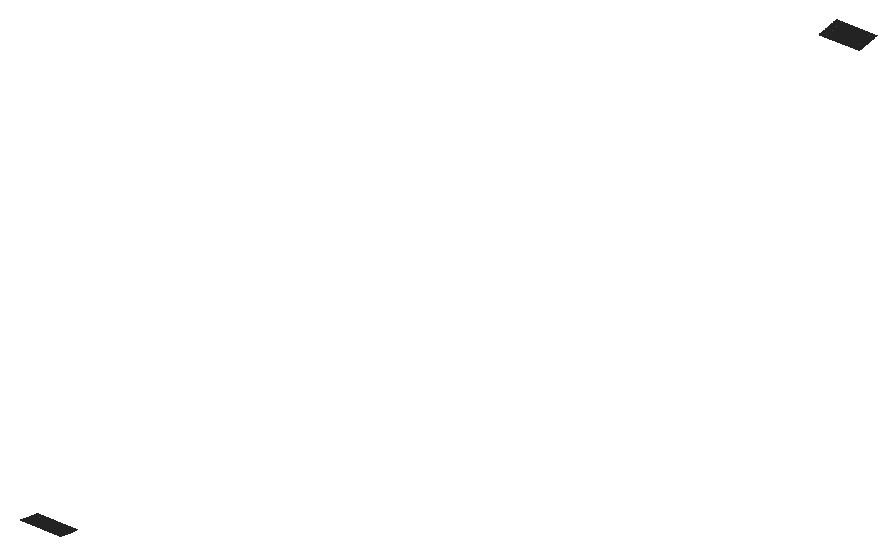
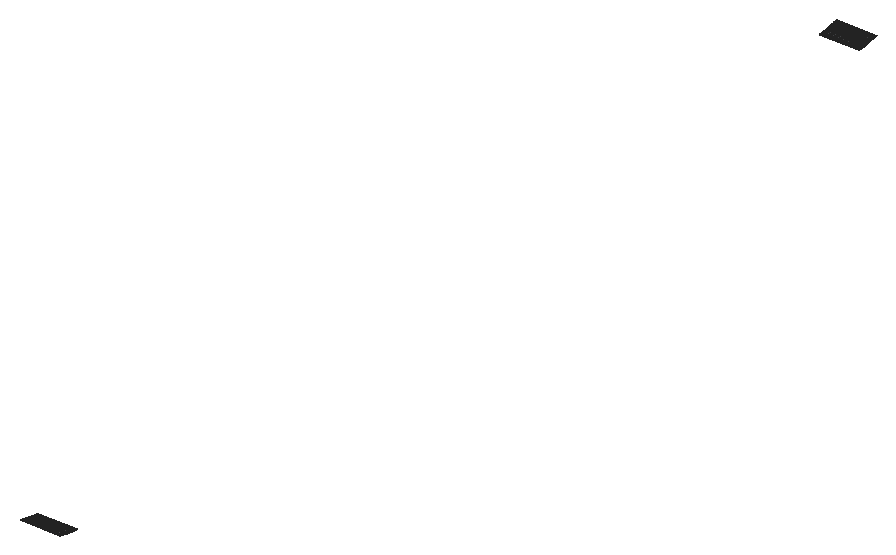
# SketchUp Ruby script. Lengths in inches.
U = 1.inch
M = Sketchup.active_model
def pt(a) = Geom::Point3d.new(a.map { |v| v * U })
def face(e, loops, mat)
  f = e.add_face(loops[0].map { |a| pt(a) })
  loops[1..].each { |l| e.add_face(l.map { |a| pt(a) }).erase! }
  f.material = f.back_material = mat if mat
  f
end
# faces: each face lists its corners as indices into pts; further lists are holes
def faces(e, pts, list, mat = nil) = list.each { |f| face(e, (f[0].is_a?(Array) ? f : [f]).map { |l| l.map { |i| pts[i] } }, mat) }
# xy, xz, yz: faces in a plane at the given z, y or x. An outline is a flat list of corners, or four numbers for a rectangle; further outlines are holes
def ring(l) = l.size == 4 ? [[l[0], l[1]], [l[2], l[1]], [l[2], l[3]], [l[0], l[3]]] : l.each_slice(2).to_a
def flat(e, list, mat, &to3) = list.each { |f| face(e, (f[0].is_a?(Array) ? f : [f]).map { |l| ring(l).map { |u, v| to3.(u, v) } }, mat) }
def xy(e, z, list, mat = nil) = flat(e, list, mat) { |x, y| [x, y, z] }
def xz(e, y, list, mat = nil) = flat(e, list, mat) { |x, z| [x, y, z] }
def yz(e, x, list, mat = nil) = flat(e, list, mat) { |y, z| [x, y, z] }
def lines(e, pts, list) = list.each { |a, b| e.add_line(pt(pts[a]), pt(pts[b])) }
# prism: a flat outline (further loops are holes) pulled along v
def prism(e, loops, v, mat = nil)
  f = face(e, loops, mat); d = Geom::Vector3d.new(v.map { |x| x * U })
  f.pushpull(f.normal.samedirection?(d) ? d.length : -d.length)
end
def box(e, o, s, mat = nil) = prism(e, [[o, [o[0] + s[0], o[1], o[2]], [o[0] + s[0], o[1] + s[1], o[2]], [o[0], o[1] + s[1], o[2]]]], [0, 0, s[2]], mat)
def at(x, y, z, deg = 0) = Geom::Transformation.translation(pt([x, y, z])) * Geom::Transformation.rotation(ORIGIN, Z_AXIS, deg.degrees)
def axes(o, x, y, z) = Geom::Transformation.new([*x, 0, *y, 0, *z, 0, *pt(o).to_a, 1])
def part(name) = M.definitions.add(name)
# library, detail: a bought-in or finely detailed component or shape, given as its bounding box
def library(name, o, s) = part(name).tap { |d| box(d.entities, o, s) }
def detail(e, o, s) = box(e.add_group.entities, o, s)
def put(e, d, t, mat = nil) = e.add_instance(d, t).tap { |i| i.material = mat if mat }
def group(e, t, mat = nil) = e.add_group.tap { |g| g.transformation = t; g.material = mat if mat }.entities
root = M.entities
M.materials.add("1432 AP 8245 TAR ROAD").color = [71, 72, 75]
p = [[573,139.98,143.95],[573,140.26,143.93],[585,140.26,143.93],[585,139.98,143.95],[573,140.55,143.9],[585,140.55,143.9],
  [573,434.48,143.93],[573,434.76,143.95],[585,434.76,143.95],[585,434.48,143.93],[573,138.86,144.08],[573,139.14,144.04],
  [585,139.14,144.04],[585,138.86,144.08],[573,139.42,144.01],[585,139.42,144.01],[573,139.7,143.98],[585,139.7,143.98],
  [573,435.04,143.98],[585,435.04,143.98],[573,435.32,144.01],[585,435.32,144.01],[573,435.6,144.04],[585,435.6,144.04],
  [573,435.88,144.08],[585,435.88,144.08],[573,138.3,144.15],[573,138.58,144.11],[585,138.58,144.11],[585,138.3,144.15],
  [573,436.16,144.11],[585,436.16,144.11],[573,436.44,144.15],[585,436.44,144.15],[573,137.46,144.28],[573,137.74,144.24],
  [585,137.74,144.24],[585,137.46,144.28],[573,138.02,144.19],[585,138.02,144.19],[573,436.72,144.19],[585,436.72,144.19],
  [573,437,144.24],[585,437,144.24],[573,437.28,144.28],[585,437.28,144.28],[573,136.9,144.38],[573,137.18,144.33],
  [585,137.18,144.33],[585,136.9,144.38],[573,437.56,144.33],[585,437.56,144.33],[573,437.84,144.38],[585,437.84,144.38],
  [573,136.35,144.48],[573,136.625,144.43],[585,136.625,144.43],[585,136.35,144.48],[573,438.12,144.43],[585,438.12,144.43],
  [573,438.39,144.48],[585,438.39,144.48],[573,135.79,144.6],[573,136.07,144.54],[585,136.07,144.54],[585,135.79,144.6],
  [573,438.67,144.54],[585,438.67,144.54],[573,438.95,144.6],[585,438.95,144.6],[573,135.52,144.66],[585,135.52,144.66],
  [573,439.22,144.66],[585,439.22,144.66],[573,134.97,144.79],[573,135.24,144.72],[585,135.24,144.72],[585,134.97,144.79],
  [573,439.5,144.72],[585,439.5,144.72],[573,439.77,144.79],[585,439.77,144.79],[573,134.69,144.85],[585,134.69,144.85],
  [573,440.05,144.85],[585,440.05,144.85],[573,134.14,144.99],[573,134.42,144.92],[585,134.42,144.92],[585,134.14,144.99],
  [573,440.32,144.92],[585,440.32,144.92],[573,440.6,144.99],[585,440.6,144.99],[573,440.87,145.07],[585,440.87,145.07]]
faces(root,p,[[0,1,2,3],[1,4,5,2],[6,7,8,9],[10,11,12,13],[11,14,15,12],[14,16,17,15],[16,0,3,17],[7,18,19,8],
  [18,20,21,19],[20,22,23,21],[22,24,25,23],[26,27,28,29],[27,10,13,28],[24,30,31,25],[30,32,33,31],[34,35,36,37],
  [35,38,39,36],[38,26,29,39],[32,40,41,33],[40,42,43,41],[42,44,45,43],[46,47,48,49],[47,34,37,48],[44,50,51,45],
  [50,52,53,51],[54,55,56,57],[55,46,49,56],[52,58,59,53],[58,60,61,59],[62,63,64,65],[63,54,57,64],[60,66,67,61],
  [66,68,69,67],[70,62,65,71],[68,72,73,69],[74,75,76,77],[75,70,71,76],[72,78,79,73],[78,80,81,79],[82,74,77,83],
  [80,84,85,81],[86,87,88,89],[87,82,83,88],[84,90,91,85],[90,92,93,91],[92,94,95,93]],"1432 AP 8245 TAR ROAD")
